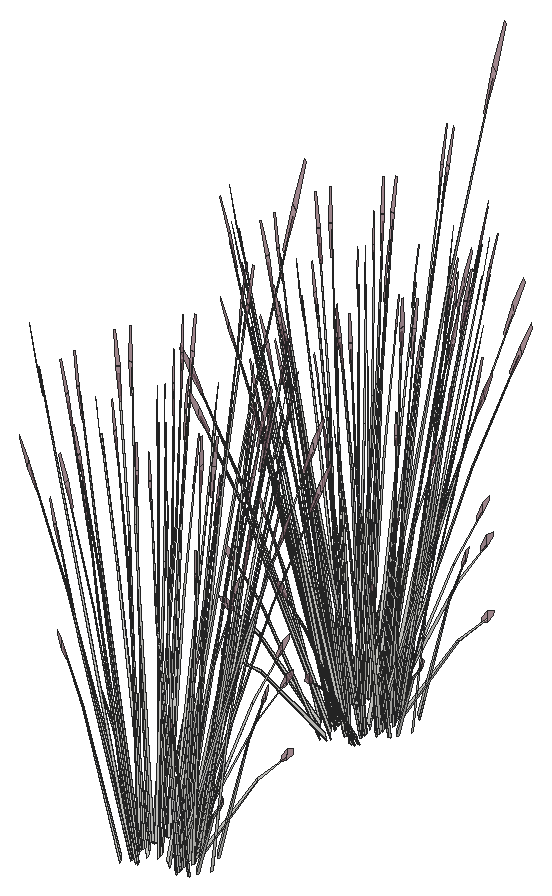
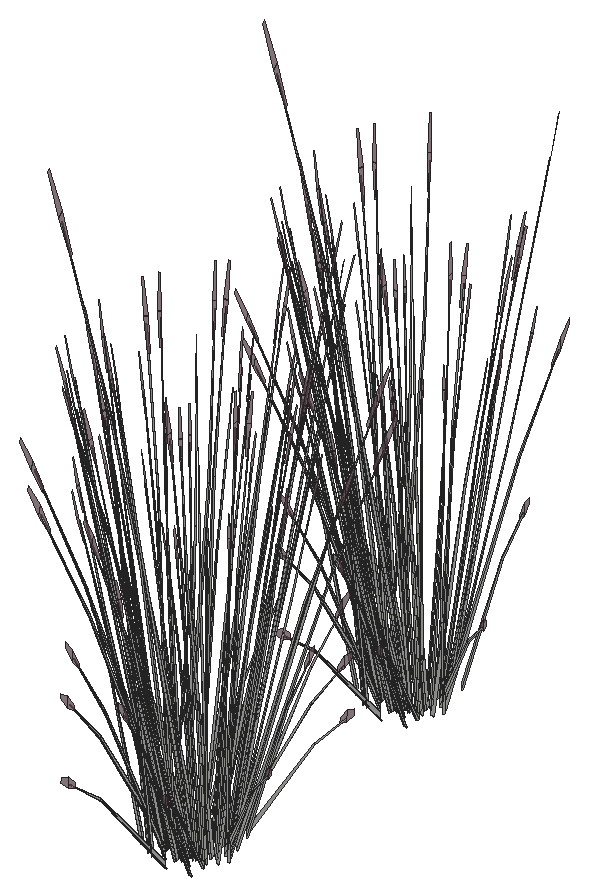
# SketchUp Ruby script. Lengths in inches.
U = 1.inch
M = Sketchup.active_model
def pt(a) = Geom::Point3d.new(a.map { |v| v * U })
def face(e, loops, mat)
  f = e.add_face(loops[0].map { |a| pt(a) })
  loops[1..].each { |l| e.add_face(l.map { |a| pt(a) }).erase! }
  f.material = f.back_material = mat if mat
  f
end
# faces: each face lists its corners as indices into pts; further lists are holes
def faces(e, pts, list, mat = nil) = list.each { |f| face(e, (f[0].is_a?(Array) ? f : [f]).map { |l| l.map { |i| pts[i] } }, mat) }
# xy, xz, yz: faces in a plane at the given z, y or x. An outline is a flat list of corners, or four numbers for a rectangle; further outlines are holes
def ring(l) = l.size == 4 ? [[l[0], l[1]], [l[2], l[1]], [l[2], l[3]], [l[0], l[3]]] : l.each_slice(2).to_a
def flat(e, list, mat, &to3) = list.each { |f| face(e, (f[0].is_a?(Array) ? f : [f]).map { |l| ring(l).map { |u, v| to3.(u, v) } }, mat) }
def xy(e, z, list, mat = nil) = flat(e, list, mat) { |x, y| [x, y, z] }
def xz(e, y, list, mat = nil) = flat(e, list, mat) { |x, z| [x, y, z] }
def yz(e, x, list, mat = nil) = flat(e, list, mat) { |y, z| [x, y, z] }
def lines(e, pts, list) = list.each { |a, b| e.add_line(pt(pts[a]), pt(pts[b])) }
# prism: a flat outline (further loops are holes) pulled along v
def prism(e, loops, v, mat = nil)
  f = face(e, loops, mat); d = Geom::Vector3d.new(v.map { |x| x * U })
  f.pushpull(f.normal.samedirection?(d) ? d.length : -d.length)
end
def box(e, o, s, mat = nil) = prism(e, [[o, [o[0] + s[0], o[1], o[2]], [o[0] + s[0], o[1] + s[1], o[2]], [o[0], o[1] + s[1], o[2]]]], [0, 0, s[2]], mat)
def at(x, y, z, deg = 0) = Geom::Transformation.translation(pt([x, y, z])) * Geom::Transformation.rotation(ORIGIN, Z_AXIS, deg.degrees)
def axes(o, x, y, z) = Geom::Transformation.new([*x, 0, *y, 0, *z, 0, *pt(o).to_a, 1])
def part(name) = M.definitions.add(name)
# library, detail: a bought-in or finely detailed component or shape, given as its bounding box
def library(name, o, s) = part(name).tap { |d| box(d.entities, o, s) }
def detail(e, o, s) = box(e.add_group.entities, o, s)
def put(e, d, t, mat = nil) = e.add_instance(d, t).tap { |i| i.material = mat if mat }
def group(e, t, mat = nil) = e.add_group.tap { |g| g.transformation = t; g.material = mat if mat }.entities
root = M.entities
M.materials.add("LightPink_Translucent").color = [144, 107, 117]
M.materials["LightPink_Translucent"].alpha = 0.75
c1 = part("blade")
p = [[2.15,0.21,22],[0,0.17,0],[0.09,0.45,0],[2.18,0.31,22],[2.29,0.31,22],[0.38,0.45,0],
  [2.48,0.24,33],[2.49,0.24,33],[2.48,0.22,33]]
faces(c1.entities,p,[[0,1,2,3],[4,5,2,3],[6,3,4,7],[8,0,3,6]])
c2 = part("seeds")
p = [[0.3,-0.1,1.38],[-0.01,-0.03,1.59],[-0.01,-0.03,0.03],[0.14,-0.07,-0.07],[0.29,-0.03,3],[0.15,0.01,3.11]]
faces(c2.entities,p,[[0,1,2,3],[1,0,4,5]],"LightPink_Translucent")
c3 = part("blade with seeds")
put(c3.entities,c1,at(0,0,0))
put(c3.entities,c2,axes([2.4,0.25,30.99],[1.5799,-0.05474,1.17369],[-0.12525,1.92788,0.29478],[-0.07173,-0.02425,1.56792]))
put(root,c3,axes([402.11,326.68,2.33],[-0.34807,-0.30426,-0.10458],[0.20053,-0.44063,-0.58045],[0.09834,-0.15317,0.88199]))
put(root,c3,axes([399.99,325.33,2.34],[0.05812,0.44446,0.30456],[-0.33222,0.11736,-0.39319],[-0.08923,-0.12737,0.75234]))
put(root,c3,axes([398.99,325.62,2.38],[0.31075,-0.40722,0.46236],[0.268,0.43246,0.38124],[-0.14579,-0.07512,0.95674]))
put(root,c3,axes([402.96,326.55,2.05],[-0.04915,-0.00419,1.5255],[-0.20409,-0.44904,-0.14414],[0.08196,-0.14765,0.26996]))
put(root,c3,axes([399.13,325.62,2.07],[0.01895,-0.4196,0.0553],[0.28611,0.0115,0.43534],[-0.1096,-0.04391,0.66383]))
put(root,c3,axes([401.9375,326.64,2.34],[-0.32754,0.07886,0.30456],[-0.08649,-0.45081,-0.39319],[0.09386,-0.12109,0.75234]))
put(root,c3,axes([402.23,326.57,2.07],[0.25832,0.23207,0.0553],[-0.1504,0.33047,0.43534],[0.08282,-0.10684,0.66383]))
put(root,c3,axes([402.16,326.47,2.07],[0.09332,0.50785,0.41282],[-0.36608,0.08814,0.34039],[0.10789,-0.11944,0.85423]))
put(root,c3,axes([403.15,327.08,2.05],[0.05222,-0.08405,1.50452],[-0.06683,-0.51557,-0.23794],[0.13101,-0.09775,0.12066]))
put(root,c3,axes([398.74,325.07,2.05],[0.0279,0.05507,1.5255],[-0.13448,0.49501,-0.14414],[-0.1362,0.00358,0.26996]))
put(root,c3,axes([399.32,325.93,2.34],[0.2141,0.34548,0.30456],[-0.24447,0.32704,-0.39319],[-0.12421,-0.04976,0.75234]))
put(root,c3,axes([399.27,325.71,2.33],[-0.02015,0.56117,-0.10458],[-0.38148,-0.01534,-0.58045],[-0.14692,-0.03898,0.88199]))
put(root,c3,axes([402.12,327.87,2.33],[-0.18933,-0.49965,-0.10458],[0.33602,-0.24554,-0.58045],[0.1416,-0.06592,0.88199]))
put(root,c3,axes([398.78,326.49,1.33],[0.15608,-0.0125,1.47384],[-0.10354,0.54165,0.11917],[-0.22242,-0.0335,0.63005]))
put(root,c3,axes([401.99,327.72,2.34],[-0.31272,-0.15393,0.30456],[0.09121,-0.44909,-0.39319],[0.1259,-0.04118,0.75234]))
put(root,c3,axes([398.72,326.9,2.07],[0.10631,-0.50312,0.41282],[0.34951,0.17204,0.34039],[-0.13745,0.03024,0.85423]))
put(root,c3,axes([398.6875,326.76,2.07],[-0.1382,-0.37624,0.0553],[0.25202,-0.18416,0.43534],[-0.11109,0.03633,0.66383]))
put(root,c3,axes([401.47,327.11,1.33],[-0.15608,0.0125,1.47384],[0.10354,-0.54165,0.11917],[0.22242,0.0335,0.63005]))
put(root,c3,axes([402.27,327.86,2.07],[0.1382,0.37624,0.0553],[-0.25202,0.18416,0.43534],[0.11109,-0.03633,0.66383]))
put(root,c3,axes([402.25,327.72,2.07],[-0.10631,0.50312,0.41282],[-0.34951,-0.17204,0.34039],[0.13745,-0.03024,0.85423]))
put(root,c3,axes([398.97,326.9,2.34],[0.31272,0.15393,0.30456],[-0.09121,0.44909,-0.39319],[-0.1259,0.04118,0.75234]))
put(root,c3,axes([402.875,329.35,2.05],[-0.03403,-0.04831,1.5255],[0.07443,-0.51782,-0.14414],[0.13402,-0.03308,0.26996]))
put(root,c3,axes([398.45,327.25,2.05],[-0.06145,0.07164,1.50452],[0.00523,0.52344,-0.23794],[-0.14085,0.06807,0.12066]))
put(root,c3,axes([398.84,326.75,2.33],[0.18933,0.49965,-0.10458],[-0.33602,0.24554,-0.58045],[-0.1416,0.06592,0.88199]))
put(root,c3,axes([402.58,328.92,1.38],[-0.07202,-0.46385,-0.03003],[0.3404,-0.10664,-0.13615],[0.07108,0.02941,0.44908]))
put(root,c3,axes([401.7,328.9,2.33],[0.02015,-0.56117,-0.10458],[0.38148,0.01534,-0.58045],[0.14692,0.03898,0.88199]))
put(root,c3,axes([401.64,328.69,2.34],[-0.2141,-0.34548,0.30456],[0.24447,-0.32704,-0.39319],[0.12421,0.04976,0.75234]))
put(root,c3,axes([402.03,328.57,2.05],[0.08072,-0.00933,1.50452],[0.22141,-0.42869,-0.23794],[0.14358,0.05659,0.12066]))
put(root,c3,axes([398.8,328.15,2.07],[-0.09332,-0.50785,0.41282],[0.36608,-0.08814,0.34039],[-0.10789,0.11944,0.85423]))
put(root,c3,axes([398.73,328.05,2.07],[-0.25832,-0.23207,0.0553],[0.1504,-0.33047,0.43534],[-0.08282,0.10684,0.66383]))
put(root,c3,axes([398.85,327.4375,1.33],[0.13056,-0.11672,1.47384],[0.10992,0.53933,0.11917],[-0.20497,0.12189,0.63005]))
put(root,c3,axes([399.02,327.98,2.34],[0.32754,-0.07886,0.30456],[0.08649,0.45081,-0.39319],[-0.09386,0.12109,0.75234]))
put(root,c3,axes([397.76,327.78,2.05],[0.04802,0.0148,1.5255],[0.14856,0.48754,-0.14414],[-0.0983,0.12796,0.26996]))
put(root,c3,axes([401.83,329,2.07],[-0.01895,0.4196,0.0553],[-0.28611,-0.0115,0.43534],[0.1096,0.04391,0.66383]))
put(root,c3,axes([401.86,328.86,2.07],[-0.27746,0.36359,0.41282],[-0.23929,-0.38612,0.34039],[0.13017,0.06707,0.85423]))
put(root,c3,axes([398.28,329.26,2.86],[0.33205,0.14729,-0.05579],[-0.10214,0.45334,-0.25298],[-0.05431,0.06883,0.83441]))
put(root,c3,axes([400.98,329.29,2.34],[-0.05812,-0.44446,0.30456],[0.33222,-0.11736,-0.39319],[0.08923,0.12737,0.75234]))
put(root,c3,axes([401.17,327.98,1.33],[-0.13977,-0.09507,1.47384],[0.28925,-0.39884,0.11917],[0.18028,0.17992,0.63005]))
put(root,c3,axes([401.2,326.73,1.85],[-0.32515,-0.2867,1.18923],[0.34333,-0.44639,0.51312],[0.10491,0.26901,1.1495]))
put(root,c3,axes([398.85,327.9375,2.33],[0.34807,0.30426,-0.10458],[-0.20053,0.44063,-0.58045],[-0.09834,0.15317,0.88199]))
put(root,c3,axes([400.94,329.52,2.33],[0.22423,-0.47232,-0.10458],[0.32472,0.27211,-0.58045],[0.11288,0.13344,0.88199]))
put(root,c3,axes([399.32,327.8,1.33],[0.09398,-0.16955,1.47384],[0.23731,0.45764,0.11917],[-0.16276,0.20841,0.63005]))
put(root,c3,axes([399.47,328.88,2.34],[0.2546,-0.29052,0.30456],[0.24101,0.33173,-0.39319],[-0.03667,0.16855,0.75234]))
put(root,c3,axes([400.65,329.91,2.05],[0.00111,-0.06681,1.5255],[0.32247,-0.29474,-0.14414],[0.11201,0.1052,0.26996]))
put(root,c3,axes([399.24,329.14,2.07],[-0.30922,-0.02571,0.0553],[0.00848,-0.38824,0.43534],[-0.03236,0.14872,0.66383]))
put(root,c3,axes([399.33,329.18,2.07],[-0.26795,-0.37649,0.41282],[0.28456,-0.3247,0.34039],[-0.04943,0.17664,0.85423]))
put(root,c3,axes([400.18,329.36,2.34],[0.11344,-0.42434,0.30456],[0.33096,0.12377,-0.39319],[0.03035,0.17085,0.75234]))
put(root,c3,axes([401.03,329.6875,2.07],[-0.17102,0.35053,0.0553],[-0.24354,-0.20408,0.43534],[0.07874,0.11238,0.66383]))
put(root,c3,axes([400.625,330.87,2.86],[0.26003,-0.31656,-0.05579],[0.23826,0.3467,-0.25298],[0.01677,0.09824,0.83441]))
put(root,c3,axes([401.1,329.59,2.07],[-0.37426,0.12663,0.41282],[-0.06495,-0.49674,0.34039],[0.08802,0.1464,0.85423]))
put(root,c3,axes([399.25,328.22,1.33],[0.07006,-0.18966,1.47384],[0.29392,0.3925,0.11917],[-0.13259,0.24463,0.63005]))
put(root,c3,axes([400.08,329.74,2.07],[-0.27727,0.18753,0.0553],[-0.13571,-0.34197,0.43534],[0.02678,0.15075,0.66383]))
put(root,c3,axes([398.46,329.2,2.05],[-0.00935,0.1092,1.50452],[0.26544,0.37987,-0.23794],[-0.06949,0.17964,0.12066]))
put(root,c3,axes([399.3,328.96,2.64],[0.41355,0.02734,-0.11608],[-0.0113,0.51765,-0.6443],[-0.02873,0.19937,0.97901]))
put(root,c3,axes([400.07,329.53,2.33],[0.36822,-0.25691,-0.10458],[0.18095,0.45596,-0.58045],[0.04858,0.19215,0.88199]))
put(root,c3,axes([400.18,329.7,2.35],[-0.37078,-0.14426,0.45823],[0.12679,-0.47426,0.37783],[0.02228,0.18651,0.9482]))
put(root,c3,axes([400.6,328.53,1.33],[-0.08601,-0.17716,1.47384],[0.39746,-0.14915,0.11917],[0.08983,0.27813,0.63005]))
put(root,c3,axes([398.43,330.32,2.05],[0.04269,-0.03331,1.5255],[0.35284,0.2216,-0.14414],[-0.00829,0.1845,0.26996]))
put(root,c3,axes([399.89,328.62,1.33],[-0.00921,-0.21179,1.47384],[0.39917,0.1405,0.11917],[-0.02469,0.30182,0.63005]))
put(root,c3,axes([399.98,330.55,2.05],[0.0477,0.08886,1.50452],[0.38493,0.03491,-0.23794],[0.03871,0.19596,0.12066]))
put(root,c3,axes([398.49,345.22,1.33],[0.08601,0.17716,1.47384],[-0.39746,0.14915,0.11917],[-0.08983,-0.27813,0.63005]))
put(root,c3,axes([399.15,344.04,2.05],[-0.05755,-0.07737,1.50452],[-0.38409,0.04905,-0.23794],[-0.0613,-0.18505,0.12066]))
put(root,c3,axes([400.87,344.99,2.05],[-0.00363,-0.10982,1.50452],[-0.30678,-0.3174,-0.23794],[0.04743,-0.1924,0.12066]))
put(root,c3,axes([399.83,345.53,1.33],[-0.07006,0.18966,1.47384],[-0.29392,-0.3925,0.11917],[0.13259,-0.24463,0.63005]))
put(root,c3,axes([400.79,344.6,2.05],[-0.03821,0.04215,1.5255],[-0.37441,-0.1422,-0.14414],[-0.01355,-0.18393,0.26996]))
put(root,c3,axes([398.75,343.79,2.05],[-0.00702,0.06614,1.5255],[-0.34622,0.24004,-0.14414],[-0.10188,-0.1227,0.26996]))
put(root,c3,axes([398.68,344.96,2.38],[0.41917,-0.14183,0.46236],[0.07275,0.55635,0.38124],[-0.09858,-0.16397,0.95674]))
put(root,c3,axes([399.625,345.07,2.07],[0.37078,0.14426,0.41282],[-0.12679,0.47426,0.34039],[-0.02228,-0.18651,0.85423]))
put(root,c3,axes([399.73,345.24,2.33],[-0.36822,0.25691,-0.10458],[-0.18095,-0.45596,-0.58045],[-0.04858,-0.19215,0.88199]))
put(root,c3,axes([400.5,345.8125,2.33],[-0.41355,-0.02734,-0.10458],[0.0113,-0.51765,-0.58045],[0.02873,-0.19937,0.88199]))
put(root,c3,axes([399.72,345.03,2.07],[0.27727,-0.18753,0.0553],[0.13571,0.34197,0.43534],[-0.02678,-0.15075,0.66383]))
put(root,c3,axes([398.77,345.08,2.07],[0.17102,-0.35053,0.0553],[0.24354,0.20408,0.43534],[-0.07874,-0.11238,0.66383]))
put(root,c3,axes([397.91,345.77,1.33],[0.13977,0.09507,1.47384],[-0.28925,0.39884,0.11917],[-0.18028,-0.17992,0.63005]))
put(root,c3,axes([399.62,345.41,2.34],[-0.11344,0.42434,0.30456],[-0.33096,-0.12377,-0.39319],[-0.03035,-0.17085,0.75234]))
put(root,c3,axes([400.47,345.59,2.07],[0.26795,0.37649,0.41282],[-0.28456,0.3247,0.34039],[0.04943,-0.17664,0.85423]))
put(root,c3,axes([398.85,345.05,2.67],[-0.25113,0.52899,-0.11713],[-0.36369,-0.30476,-0.65011],[-0.12642,-0.14945,0.98783]))
put(root,c3,axes([400.5625,345.63,2.07],[0.30922,0.02571,0.0553],[-0.00848,0.38824,0.43534],[0.03236,-0.14872,0.66383]))
put(root,c3,axes([400.33,345.89,2.34],[-0.2546,0.29052,0.30456],[-0.24101,-0.33173,-0.39319],[0.03667,-0.16855,0.75234]))
put(root,c3,axes([397.89,344.89,2.05],[-0.08096,-0.00389,1.50452],[-0.25776,0.38949,-0.23794],[-0.13753,-0.07958,0.12066]))
put(root,c3,axes([400.95,346.83,2.33],[-0.34807,-0.30426,-0.10458],[0.20053,-0.44063,-0.58045],[0.09834,-0.15317,0.88199]))
put(root,c3,axes([398.83,345.49,2.34],[0.05812,0.44446,0.30456],[-0.33222,0.11736,-0.39319],[-0.08923,-0.12737,0.75234]))
put(root,c3,axes([397.83,345.77,2.38],[0.31075,-0.40722,0.46236],[0.268,0.43246,0.38124],[-0.14579,-0.07512,0.95674]))
put(root,c3,axes([401.8,346.7,2.05],[-0.04915,-0.00419,1.5255],[-0.20409,-0.44904,-0.14414],[0.08196,-0.14765,0.26996]))
put(root,c3,axes([397.97,345.77,2.07],[0.01895,-0.4196,0.0553],[0.28611,0.0115,0.43534],[-0.1096,-0.04391,0.66383]))
put(root,c3,axes([400.78,346.79,2.34],[-0.32754,0.07886,0.30456],[-0.08649,-0.45081,-0.39319],[0.09386,-0.12109,0.75234]))
put(root,c3,axes([401.07,346.72,2.07],[0.25832,0.23207,0.0553],[-0.1504,0.33047,0.43534],[0.08282,-0.10684,0.66383]))
put(root,c3,axes([401,346.62,2.07],[0.09332,0.50785,0.41282],[-0.36608,0.08814,0.34039],[0.10789,-0.11944,0.85423]))
put(root,c3,axes([401.99,347.24,2.05],[0.05222,-0.08405,1.50452],[-0.06683,-0.51557,-0.23794],[0.13101,-0.09775,0.12066]))
put(root,c3,axes([397.58,345.22,2.05],[0.0279,0.05507,1.5255],[-0.13448,0.49501,-0.14414],[-0.1362,0.00358,0.26996]))
put(root,c3,axes([398.16,346.09,2.34],[0.2141,0.34548,0.30456],[-0.24447,0.32704,-0.39319],[-0.12421,-0.04976,0.75234]))
put(root,c3,axes([398.1,345.87,2.33],[-0.02015,0.56117,-0.10458],[-0.38148,-0.01534,-0.58045],[-0.14692,-0.03898,0.88199]))
put(root,c3,axes([400.96,348.02,2.33],[-0.18933,-0.49965,-0.10458],[0.33602,-0.24554,-0.58045],[0.1416,-0.06592,0.88199]))
put(root,c3,axes([397.62,346.64,1.33],[0.15608,-0.0125,1.47384],[-0.10354,0.54165,0.11917],[-0.22242,-0.0335,0.63005]))
put(root,c3,axes([400.83,347.87,2.34],[-0.31272,-0.15393,0.30456],[0.09121,-0.44909,-0.39319],[0.1259,-0.04118,0.75234]))
put(root,c3,axes([397.55,347.05,2.07],[0.10631,-0.50312,0.41282],[0.34951,0.17204,0.34039],[-0.13745,0.03024,0.85423]))
put(root,c3,axes([397.53,346.91,2.07],[-0.1382,-0.37624,0.0553],[0.25202,-0.18416,0.43534],[-0.11109,0.03633,0.66383]))
put(root,c3,axes([400.31,347.26,1.33],[-0.15608,0.0125,1.47384],[0.10354,-0.54165,0.11917],[0.22242,0.0335,0.63005]))
put(root,c3,axes([401.11,348.01,2.07],[0.1382,0.37624,0.0553],[-0.25202,0.18416,0.43534],[0.11109,-0.03633,0.66383]))
put(root,c3,axes([401.08,347.875,2.07],[-0.10631,0.50312,0.41282],[-0.34951,-0.17204,0.34039],[0.13745,-0.03024,0.85423]))
put(root,c3,axes([397.8125,347.05,2.34],[0.31272,0.15393,0.30456],[-0.09121,0.44909,-0.39319],[-0.1259,0.04118,0.75234]))
put(root,c3,axes([401.71,349.5,2.05],[-0.03403,-0.04831,1.5255],[0.07443,-0.51782,-0.14414],[0.13402,-0.03308,0.26996]))
put(root,c3,axes([397.28,347.4,2.05],[-0.06145,0.07164,1.50452],[0.00523,0.52344,-0.23794],[-0.14085,0.06807,0.12066]))
put(root,c3,axes([397.68,346.9,2.33],[0.18933,0.49965,-0.10458],[-0.33602,0.24554,-0.58045],[-0.1416,0.06592,0.88199]))
put(root,c3,axes([401.42,349.07,1.38],[-0.07202,-0.46385,-0.03003],[0.3404,-0.10664,-0.13615],[0.07108,0.02941,0.44908]))
put(root,c3,axes([400.53,349.06,2.33],[0.02015,-0.56117,-0.10458],[0.38148,0.01534,-0.58045],[0.14692,0.03898,0.88199]))
put(root,c3,axes([400.48,348.84,2.34],[-0.2141,-0.34548,0.30456],[0.24447,-0.32704,-0.39319],[0.12421,0.04976,0.75234]))
put(root,c3,axes([400.87,348.72,2.05],[0.08072,-0.00933,1.50452],[0.22141,-0.42869,-0.23794],[0.14358,0.05659,0.12066]))
put(root,c3,axes([397.64,348.3,2.07],[-0.09332,-0.50785,0.41282],[0.36608,-0.08814,0.34039],[-0.10789,0.11944,0.85423]))
put(root,c3,axes([397.57,348.2,2.07],[-0.25832,-0.23207,0.0553],[0.1504,-0.33047,0.43534],[-0.08282,0.10684,0.66383]))
put(root,c3,axes([397.68,347.59,1.33],[0.13056,-0.11672,1.47384],[0.10992,0.53933,0.11917],[-0.20497,0.12189,0.63005]))
put(root,c3,axes([397.86,348.13,2.34],[0.32754,-0.07886,0.30456],[0.08649,0.45081,-0.39319],[-0.09386,0.12109,0.75234]))
put(root,c3,axes([396.6,347.93,2.05],[0.04802,0.0148,1.5255],[0.14856,0.48754,-0.14414],[-0.0983,0.12796,0.26996]))
put(root,c3,axes([400.67,349.15,2.07],[-0.01895,0.4196,0.0553],[-0.28611,-0.0115,0.43534],[0.1096,0.04391,0.66383]))
put(root,c3,axes([400.7,349.02,2.07],[-0.27746,0.36359,0.41282],[-0.23929,-0.38612,0.34039],[0.13017,0.06707,0.85423]))
put(root,c3,axes([397.12,349.41,2.86],[0.33205,0.14729,-0.05579],[-0.10214,0.45334,-0.25298],[-0.05431,0.06883,0.83441]))
put(root,c3,axes([399.8125,349.4375,2.34],[-0.05812,-0.44446,0.30456],[0.33222,-0.11736,-0.39319],[0.08923,0.12737,0.75234]))
put(root,c3,axes([400.01,348.13,1.33],[-0.13977,-0.09507,1.47384],[0.28925,-0.39884,0.11917],[0.18028,0.17992,0.63005]))
put(root,c3,axes([400.04,346.88,1.85],[-0.32515,-0.2867,1.18923],[0.34333,-0.44639,0.51312],[0.10491,0.26901,1.1495]))
put(root,c3,axes([397.69,348.09,2.33],[0.34807,0.30426,-0.10458],[-0.20053,0.44063,-0.58045],[-0.09834,0.15317,0.88199]))
put(root,c3,axes([399.78,349.67,2.33],[0.22423,-0.47232,-0.10458],[0.32472,0.27211,-0.58045],[0.11288,0.13344,0.88199]))
put(root,c3,axes([398.16,347.96,1.33],[0.09398,-0.16955,1.47384],[0.23731,0.45764,0.11917],[-0.16276,0.20841,0.63005]))
put(root,c3,axes([398.31,349.03,2.34],[0.2546,-0.29052,0.30456],[0.24101,0.33173,-0.39319],[-0.03667,0.16855,0.75234]))
put(root,c3,axes([399.49,350.06,2.05],[0.00111,-0.06681,1.5255],[0.32247,-0.29474,-0.14414],[0.11201,0.1052,0.26996]))
put(root,c3,axes([398.07,349.29,2.07],[-0.30922,-0.02571,0.0553],[0.00848,-0.38824,0.43534],[-0.03236,0.14872,0.66383]))
put(root,c3,axes([398.17,349.33,2.07],[-0.26795,-0.37649,0.41282],[0.28456,-0.3247,0.34039],[-0.04943,0.17664,0.85423]))
put(root,c3,axes([399.02,349.51,2.34],[0.11344,-0.42434,0.30456],[0.33096,0.12377,-0.39319],[0.03035,0.17085,0.75234]))
put(root,c3,axes([399.87,349.84,2.07],[-0.17102,0.35053,0.0553],[-0.24354,-0.20408,0.43534],[0.07874,0.11238,0.66383]))
put(root,c3,axes([399.46,351.02,2.86],[0.26003,-0.31656,-0.05579],[0.23826,0.3467,-0.25298],[0.01677,0.09824,0.83441]))
put(root,c3,axes([399.9375,349.74,2.07],[-0.37426,0.12663,0.41282],[-0.06495,-0.49674,0.34039],[0.08802,0.1464,0.85423]))
put(root,c3,axes([398.09,348.375,1.33],[0.07006,-0.18966,1.47384],[0.29392,0.3925,0.11917],[-0.13259,0.24463,0.63005]))
put(root,c3,axes([398.92,349.89,2.07],[-0.27727,0.18753,0.0553],[-0.13571,-0.34197,0.43534],[0.02678,0.15075,0.66383]))
put(root,c3,axes([397.29,349.36,2.05],[-0.00935,0.1092,1.50452],[0.26544,0.37987,-0.23794],[-0.06949,0.17964,0.12066]))
put(root,c3,axes([398.14,349.11,2.64],[0.41355,0.02734,-0.11608],[-0.0113,0.51765,-0.6443],[-0.02873,0.19937,0.97901]))
put(root,c3,axes([398.91,349.6875,2.33],[0.36822,-0.25691,-0.10458],[0.18095,0.45596,-0.58045],[0.04858,0.19215,0.88199]))
put(root,c3,axes([399.01,349.86,2.35],[-0.37078,-0.14426,0.45823],[0.12679,-0.47426,0.37783],[0.02228,0.18651,0.9482]))
put(root,c3,axes([399.43,348.6875,1.33],[-0.08601,-0.17716,1.47384],[0.39746,-0.14915,0.11917],[0.08983,0.27813,0.63005]))
put(root,c3,axes([397.26,350.48,2.05],[0.04269,-0.03331,1.5255],[0.35284,0.2216,-0.14414],[-0.00829,0.1845,0.26996]))
put(root,c3,axes([398.73,348.77,1.33],[-0.00921,-0.21179,1.47384],[0.39917,0.1405,0.11917],[-0.02469,0.30182,0.63005]))
put(root,c3,axes([398.82,350.71,2.05],[0.0477,0.08886,1.50452],[0.38493,0.03491,-0.23794],[0.03871,0.19596,0.12066]))
